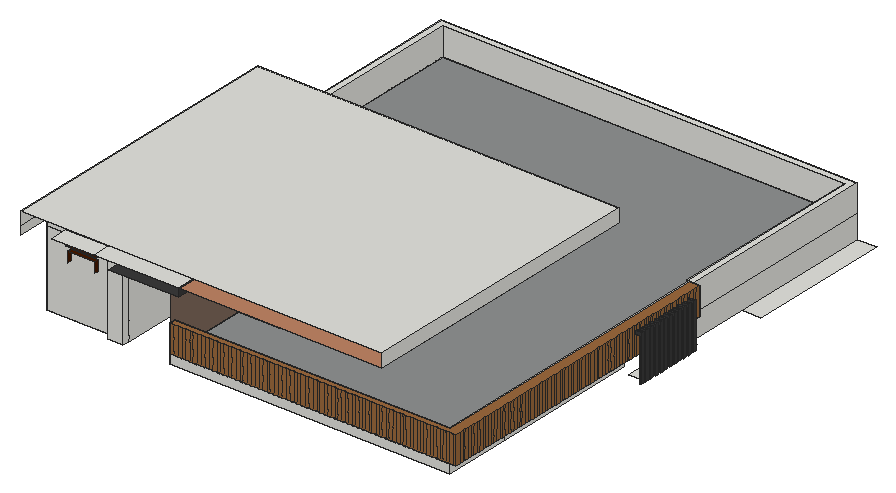
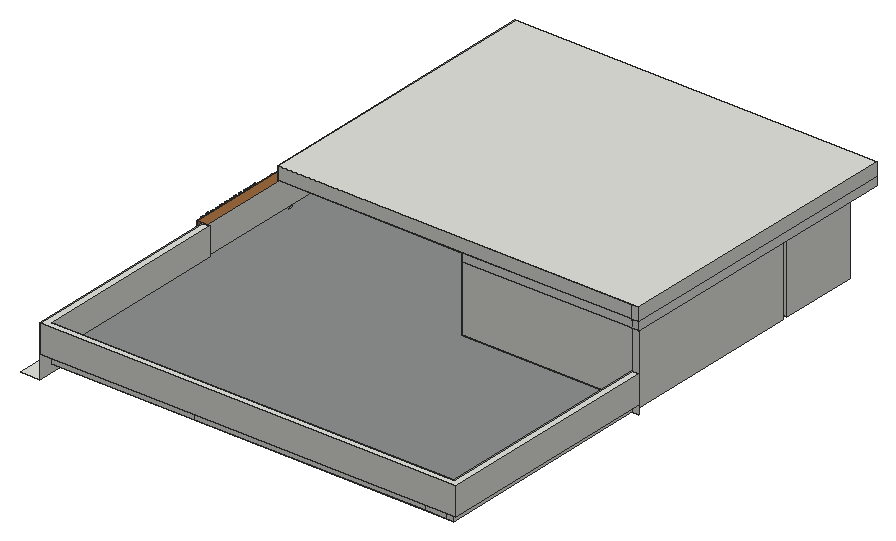
# SketchUp Ruby script. Lengths in inches.
U = 1.inch
M = Sketchup.active_model
def pt(a) = Geom::Point3d.new(a.map { |v| v * U })
def face(e, loops, mat)
  f = e.add_face(loops[0].map { |a| pt(a) })
  loops[1..].each { |l| e.add_face(l.map { |a| pt(a) }).erase! }
  f.material = f.back_material = mat if mat
  f
end
# faces: each face lists its corners as indices into pts; further lists are holes
def faces(e, pts, list, mat = nil) = list.each { |f| face(e, (f[0].is_a?(Array) ? f : [f]).map { |l| l.map { |i| pts[i] } }, mat) }
# xy, xz, yz: faces in a plane at the given z, y or x. An outline is a flat list of corners, or four numbers for a rectangle; further outlines are holes
def ring(l) = l.size == 4 ? [[l[0], l[1]], [l[2], l[1]], [l[2], l[3]], [l[0], l[3]]] : l.each_slice(2).to_a
def flat(e, list, mat, &to3) = list.each { |f| face(e, (f[0].is_a?(Array) ? f : [f]).map { |l| ring(l).map { |u, v| to3.(u, v) } }, mat) }
def xy(e, z, list, mat = nil) = flat(e, list, mat) { |x, y| [x, y, z] }
def xz(e, y, list, mat = nil) = flat(e, list, mat) { |x, z| [x, y, z] }
def yz(e, x, list, mat = nil) = flat(e, list, mat) { |y, z| [x, y, z] }
def lines(e, pts, list) = list.each { |a, b| e.add_line(pt(pts[a]), pt(pts[b])) }
# prism: a flat outline (further loops are holes) pulled along v
def prism(e, loops, v, mat = nil)
  f = face(e, loops, mat); d = Geom::Vector3d.new(v.map { |x| x * U })
  f.pushpull(f.normal.samedirection?(d) ? d.length : -d.length)
end
def box(e, o, s, mat = nil) = prism(e, [[o, [o[0] + s[0], o[1], o[2]], [o[0] + s[0], o[1] + s[1], o[2]], [o[0], o[1] + s[1], o[2]]]], [0, 0, s[2]], mat)
def at(x, y, z, deg = 0) = Geom::Transformation.translation(pt([x, y, z])) * Geom::Transformation.rotation(ORIGIN, Z_AXIS, deg.degrees)
def axes(o, x, y, z) = Geom::Transformation.new([*x, 0, *y, 0, *z, 0, *pt(o).to_a, 1])
def part(name) = M.definitions.add(name)
# library, detail: a bought-in or finely detailed component or shape, given as its bounding box
def library(name, o, s) = part(name).tap { |d| box(d.entities, o, s) }
def detail(e, o, s) = box(e.add_group.entities, o, s)
def put(e, d, t, mat = nil) = e.add_instance(d, t).tap { |i| i.material = mat if mat }
def group(e, t, mat = nil) = e.add_group.tap { |g| g.transformation = t; g.material = mat if mat }.entities
root = M.entities
M.materials.add("[Blacktop Old 02]").color = [143, 145, 145]
M.materials.add("[Color B08]").color = [69, 25, 0]
M.materials.add("[Color E01]").color = [255, 255, 204]
M.materials.add("[Color M07]").color = [58, 58, 58]
M.materials.add("[Granite Brown]").color = [126, 104, 91]
M.materials.add("[Modern Siding]").color = [191, 132, 100]
M.materials.add("[Wood Floor]").color = [155, 105, 61]
xy(root,515.86,[[540,499.48,564.9375,687]])
xy(root,516.1,[[554.5,316.14,556.8125,319.52],[554.5,323.77,556.8125,327.14],[554.5,331.39,556.8125,334.77],[554.5,339.02,556.8125,342.39],[554.5,346.64,556.8125,350.02],
  [554.5,354.27,556.8125,357.64],[554.5,361.89,556.8125,365.27],[554.5,369.52,556.8125,372.89],[554.5,377.14,556.8125,380.52],[554.5,384.77,556.8125,388.14],
  [554.5,392.39,556.8125,395.77],[554.5,400.89,556.8125,404.27]],"[Color M07]")
xy(root,521.1,[[540,316.14,554.5,408.01]])
xy(root,533.5625,[[9,36,18.8125,137.125],[18.8125,36,114.93,137.125],[345.1875,113.4375,345.1875,137.125,351.1875,137.125,351.1875,121.0625,531,121.0625,531,113.4375],[531,113.4375,531.51,137.125],[351.1875,121.0625,531,288],
  [18.8125,137.125,224.375,144.4375],[224.375,137.125,230.375,144.4375],[230.375,137.125,345.1875,144.4375],[345.1875,137.125,345.1875,294,531,294,531,288,351.1875,288,351.1875,137.125],[9,144.4375,18.8125,382.6875],
  [18.8125,144.4375,224.375,382.6875],[224.375,144.4375,224.375,382.6875,18.8125,382.6875,18.8125,388.6875,230.375,388.6875,230.375,144.4375],[230.375,144.4375,230.375,388.6875,18.8125,388.6875,18.8125,678,531,678,531,294,345.1875,294,345.1875,144.4375],[9,388.6875,18.8125,678]])
xy(root,533.5625,[[176.76,25.875,176.76,137.125,345.1875,137.125,345.1875,113.4375,540,113.4375,540,25.875]],"[Wood Floor]")
xy(root,545.5625,[[176.76,25.875,176.76,33.625,534,33.625,534,421.98,540,421.98,540,25.875],[0,388.6875,0,687,540,687,540,421.98,531,421.98,531,678,9,678,9,388.6875]])
xy(root,545.5625,[[176.76,33.625,534,33.625,534,421.98,531,421.98,531,678,9,678,9,388.6875,230.375,388.6875,230.375,137.125,176.76,137.125]],"[Blacktop Old 02]")
xy(root,545.5625,[[540,25.875,548.1875,421.98]],"[Wood Floor]")
xy(root,550.125,[[18.8125,144.4375,224.375,382.6875]])
xy(root,571.13,[[548.25,400.89,554.5,404.27]])
xy(root,571.13,[[547.5625,316.14,554.5,319.52],[548.1875,323.77,554.5,327.14],[548.1875,331.39,554.5,334.77],[548.1875,339.02,554.5,342.39],[548.1875,346.64,554.5,350.02],
  [548.1875,354.27,554.5,357.64],[548.1875,361.89,554.5,365.27],[548.1875,369.52,554.5,372.89],[548.1875,377.14,554.5,380.52],[548.1875,384.77,554.5,388.14],
  [548.1875,392.39,554.5,395.77]],"[Color M07]")
xy(root,575.41,[[548.1875,369.52,556.8125,372.89],[548.1875,377.14,556.8125,380.52],[548.1875,384.77,556.8125,388.14],[548.1875,392.39,556.8125,395.77],[548.25,400.89,556.8125,404.27]],"[Color M07]")
xy(root,575.72,[[547.5625,316.14,556.8125,319.52],[548.1875,323.77,556.8125,327.14],[548.1875,331.39,556.8125,334.77],[548.1875,339.02,556.8125,342.39],[548.1875,346.64,556.8125,350.02],
  [548.1875,354.27,556.8125,357.64],[548.1875,361.89,556.8125,365.27]],"[Color M07]")
xy(root,581.5625,[[0,388.6875,9,388.6875,9,678,531,678,531,421.98,540,421.98,540,687,0,687]])
xy(root,581.5625,[[176.76,25.875,548.1875,25.875,548.1875,421.98,534,421.98,534,33.625,176.76,33.625]],"[Wood Floor]")
xy(root,621.29,[[47.49,22.1875,82.4,27]],"[Color B08]")
xy(root,626.03,[[44.88,22.1875,85.01,27]],"[Color B08]")
xy(root,631.3125,[[94.8,27,114.93,36],[114.93,27,176.76,36],[94.8,36,114.93,137.125],[114.93,36,176.76,137.125],[94.8,137.125,205.99,144.4375],
  [94.8,144.4375,205.99,144.8125]])
xy(root,631.3125,[[114.93,3.875,114.93,27,176.76,27,176.76,137.125,205.99,137.125,205.99,3.875]],"[Color M07]")
xy(root,641.625,[[40.88,3.875,94.8,27],[94.8,3.875,205.99,36],[9,36,94.8,137.125],[94.8,36,205.99,137.125],[94.8,137.125,205.99,144.8125]])
xy(root,641.625,[[205.99,3.875,469.36,137.125],[230.375,137.125,469.36,388.6875]],"[Modern Siding]")
xy(root,658.875,[[0,3.875,469.36,388.6875]])
xz(root,25.875,[[176.76,533.5625,540,545.5625]])
xz(root,25.875,[[176.76,545.5625,181.89,581.5625],[181.89,545.5625,186.89,581.5625],[186.89,545.5625,191.89,581.5625],[191.89,545.5625,196.89,581.5625],[196.89,545.5625,201.89,581.5625],
  [201.89,545.5625,206.89,581.5625],[206.89,545.5625,211.89,581.5625],[211.89,545.5625,216.89,581.5625],[216.89,545.5625,221.89,581.5625],[221.89,545.5625,226.89,581.5625],
  [226.89,545.5625,231.89,581.5625],[231.89,545.5625,236.89,581.5625],[236.89,545.5625,241.89,581.5625],[241.89,545.5625,246.89,581.5625],[246.89,545.5625,251.89,581.5625],
  [251.89,545.5625,256.89,581.5625],[256.89,545.5625,261.89,581.5625],[261.89,545.5625,266.89,581.5625],[266.89,545.5625,271.89,581.5625],[271.89,545.5625,276.89,581.5625],
  [276.89,545.5625,281.89,581.5625],[281.89,545.5625,286.89,581.5625],[286.89,545.5625,291.89,581.5625],[291.89,545.5625,296.89,581.5625],[296.89,545.5625,301.89,581.5625],
  [301.89,545.5625,306.89,581.5625],[306.89,545.5625,311.89,581.5625],[311.89,545.5625,316.89,581.5625],[316.89,545.5625,321.89,581.5625],[321.89,545.5625,326.89,581.5625],
  [326.89,545.5625,331.89,581.5625],[331.89,545.5625,336.89,581.5625],[336.89,545.5625,341.89,581.5625],[341.89,545.5625,346.89,581.5625],[346.89,545.5625,351.89,581.5625],
  [351.89,545.5625,356.89,581.5625],[356.89,545.5625,361.89,581.5625],[361.89,545.5625,366.89,581.5625],[366.89,545.5625,371.89,581.5625],[371.89,545.5625,376.89,581.5625],
  [376.89,545.5625,381.33,581.5625],[381.33,545.5625,385.77,581.5625],[385.77,545.5625,390.2,581.5625],[390.2,545.5625,394.64,581.5625],[394.64,545.5625,399.08,581.5625],
  [399.08,545.5625,403.52,581.5625],[403.52,545.5625,407.95,581.5625],[407.95,545.5625,412.39,581.5625],[412.39,545.5625,416.83,581.5625],[416.83,545.5625,421.27,581.5625],
  [421.27,545.5625,425.7,581.5625],[425.7,545.5625,430.14,581.5625],[430.14,545.5625,434.58,581.5625],[434.58,545.5625,439.02,581.5625],[439.02,545.5625,443.45,581.5625],
  [443.45,545.5625,447.89,581.5625],[447.89,545.5625,452.33,581.5625],[452.33,545.5625,456.77,581.5625],[456.77,545.5625,461.2,581.5625],[461.2,545.5625,465.64,581.5625],
  [465.64,545.5625,470.08,581.5625],[470.08,545.5625,474.52,581.5625],[474.52,545.5625,478.95,581.5625],[478.95,545.5625,483.39,581.5625],[483.39,545.5625,487.83,581.5625],
  [487.83,545.5625,492.27,581.5625],[492.27,545.5625,496.7,581.5625],[496.7,545.5625,501.14,581.5625],[501.14,545.5625,505.58,581.5625],[505.58,545.5625,510.02,581.5625],
  [510.02,545.5625,514.2,581.5625],[514.2,545.5625,518.39,581.5625],[518.39,545.5625,522.58,581.5625],[522.58,545.5625,526.77,581.5625],[526.77,545.5625,530.95,581.5625],
  [530.95,545.5625,535.14,581.5625],[535.14,545.5625,539.33,581.5625],[539.33,545.5625,543.33,581.5625],[543.33,545.5625,548.1875,581.5625]],"[Wood Floor]")
xz(root,27,[[94.8,533.5625,114.93,631.3125]])
xz(root,33.625,[[176.76,545.5625,534,581.5625]])
xz(root,36,[[9,533.5625,114.93,631.3125],[9,631.3125,94.8,641.625]])
xz(root,137.125,[[9,533.5625,22.75,631.3125],[22.75,533.5625,114.93,631.3125],[114.93,533.5625,176.76,631.3125],[176.76,533.5625,224.375,545.5625],[224.375,533.5625,230.375,545.5625],
  [531,533.5625,531.51,545.5625],[9,631.3125,22.75,641.625],[22.75,631.3125,94.8,641.625]])
xz(root,137.125,[[176.76,545.5625,230.375,545.5625,230.375,641.625,205.99,641.625,205.99,631.3125,176.76,631.3125]],"[Color E01]")
xz(root,144.4375,[[9,533.5625,9,631.3125,224.375,631.3125,224.375,550.125,18.8125,550.125,18.8125,533.5625],[18.8125,533.5625,224.375,550.125],[9,631.3125,94.8,641.625],[205.99,631.3125,224.375,641.625]])
xz(root,144.8125,[[94.8,631.3125,205.99,641.625]])
xz(root,316.14,[[554.5,516.1,556.8125,516.1,556.8125,575.72,547.5625,575.72,547.5625,571.13,554.5,571.13]],"[Color M07]")
xz(root,319.52,[[554.5,516.1,554.5,571.13,547.5625,571.13,547.5625,575.72,556.8125,575.72,556.8125,516.1]],"[Color M07]")
xz(root,323.77,[[554.5,516.1,556.8125,516.1,556.8125,575.72,548.1875,575.72,548.1875,571.13,554.5,571.13]],"[Color M07]")
xz(root,327.14,[[554.5,516.1,554.5,571.13,548.1875,571.13,548.1875,575.72,556.8125,575.72,556.8125,516.1]],"[Color M07]")
xz(root,331.39,[[554.5,516.1,556.8125,516.1,556.8125,575.72,548.1875,575.72,548.1875,571.13,554.5,571.13]],"[Color M07]")
xz(root,334.77,[[554.5,516.1,554.5,571.13,548.1875,571.13,548.1875,575.72,556.8125,575.72,556.8125,516.1]],"[Color M07]")
xz(root,339.02,[[554.5,516.1,556.8125,516.1,556.8125,575.72,548.1875,575.72,548.1875,571.13,554.5,571.13]],"[Color M07]")
xz(root,342.39,[[554.5,516.1,554.5,571.13,548.1875,571.13,548.1875,575.72,556.8125,575.72,556.8125,516.1]],"[Color M07]")
xz(root,346.64,[[554.5,516.1,556.8125,516.1,556.8125,575.72,548.1875,575.72,548.1875,571.13,554.5,571.13]],"[Color M07]")
xz(root,350.02,[[554.5,516.1,554.5,571.13,548.1875,571.13,548.1875,575.72,556.8125,575.72,556.8125,516.1]],"[Color M07]")
xz(root,354.27,[[554.5,516.1,556.8125,516.1,556.8125,575.72,548.1875,575.72,548.1875,571.13,554.5,571.13]],"[Color M07]")
xz(root,357.64,[[554.5,516.1,554.5,571.13,548.1875,571.13,548.1875,575.72,556.8125,575.72,556.8125,516.1]],"[Color M07]")
xz(root,361.89,[[554.5,516.1,556.8125,516.1,556.8125,575.72,548.1875,575.72,548.1875,571.13,554.5,571.13]],"[Color M07]")
xz(root,365.27,[[554.5,516.1,554.5,571.13,548.1875,571.13,548.1875,575.72,556.8125,575.72,556.8125,516.1]],"[Color M07]")
xz(root,369.52,[[554.5,516.1,556.8125,516.1,556.8125,575.41,548.1875,575.41,548.1875,571.13,554.5,571.13]],"[Color M07]")
xz(root,372.89,[[554.5,516.1,554.5,571.13,548.1875,571.13,548.1875,575.41,556.8125,575.41,556.8125,516.1]],"[Color M07]")
xz(root,377.14,[[554.5,516.1,556.8125,516.1,556.8125,575.41,548.1875,575.41,548.1875,571.13,554.5,571.13]],"[Color M07]")
xz(root,380.52,[[554.5,516.1,554.5,571.13,548.1875,571.13,548.1875,575.41,556.8125,575.41,556.8125,516.1]],"[Color M07]")
xz(root,382.6875,[[9,533.5625,18.8125,533.5625,18.8125,550.125,224.375,550.125,224.375,631.3125,9,631.3125],[18.8125,533.5625,224.375,550.125],[9,631.3125,224.375,641.625]])
xz(root,384.77,[[554.5,516.1,556.8125,516.1,556.8125,575.41,548.1875,575.41,548.1875,571.13,554.5,571.13]],"[Color M07]")
xz(root,388.14,[[554.5,516.1,554.5,571.13,548.1875,571.13,548.1875,575.41,556.8125,575.41,556.8125,516.1]],"[Color M07]")
xz(root,388.6875,[[0,533.5625,9,545.5625],[9,533.5625,18.8125,545.5625],[18.8125,533.5625,230.375,545.5625],[0,545.5625,9,581.5625],[9,545.5625,230.375,631.3125],
  [0,581.5625,9,631.3125],[0,631.3125,9,641.625],[9,631.3125,230.375,641.625],[0,641.625,9,658.875],[9,641.625,469.36,658.875]])
xz(root,392.39,[[554.5,516.1,556.8125,516.1,556.8125,575.41,548.1875,575.41,548.1875,571.13,554.5,571.13]],"[Color M07]")
xz(root,395.77,[[554.5,516.1,554.5,571.13,548.1875,571.13,548.1875,575.41,556.8125,575.41,556.8125,516.1]],"[Color M07]")
xz(root,400.89,[[554.5,516.1,556.8125,516.1,556.8125,575.41,548.25,575.41,548.25,571.13,554.5,571.13]],"[Color M07]")
xz(root,404.27,[[554.5,516.1,554.5,571.13,548.25,571.13,548.25,575.41,556.8125,575.41,556.8125,516.1]],"[Color M07]")
xz(root,421.98,[[531,545.5625,534,581.5625],[534,545.5625,540,581.5625]])
xz(root,421.98,[[540,545.5625,548.1875,581.5625]],"[Wood Floor]")
xz(root,678,[[9,533.5625,18.8125,545.5625],[18.8125,533.5625,45.875,545.5625],[45.875,533.5625,345.75,545.5625],[345.75,533.5625,531,545.5625],[9,545.5625,531,581.5625]])
xz(root,687,[[0,545.5625,540,581.5625]])
yz(root,0,[[388.6875,545.5625,687,581.5625],[3.875,631.3125,388.6875,641.625],[3.875,641.625,388.6875,658.875]])
yz(root,9,[[36,533.5625,137.125,631.3125],[144.4375,533.5625,382.6875,631.3125],[388.6875,533.5625,678,545.5625],[388.6875,545.5625,678,581.5625],[36,631.3125,137.125,641.625]])
yz(root,18.8125,[[144.4375,533.5625,382.6875,550.125]])
yz(root,47.49,[[22.1875,607.67,27,621.29]],"[Color B08]")
yz(root,82.4,[[22.1875,607.67,27,621.29]],"[Color B08]")
yz(root,94.8,[[27,631.3125,36,641.625],[36,631.3125,137.125,641.625],[137.125,631.3125,144.4375,641.625],[144.4375,631.3125,144.8125,641.625],[144.4375,641.625,144.8125,648.6875]])
yz(root,114.93,[[27,533.5625,36,631.3125],[36,533.5625,137.125,631.3125]])
yz(root,176.76,[[25.875,533.5625,27,545.5625],[27,533.5625,137.125,545.5625],[25.875,545.5625,27,581.5625],[27,545.5625,33.625,581.5625]])
yz(root,176.76,[[33.625,545.5625,137.125,545.5625,137.125,631.3125,27,631.3125,27,581.5625,33.625,581.5625]],"[Granite Brown]")
yz(root,205.99,[[137.125,631.3125,144.4375,641.625],[144.4375,631.3125,144.8125,641.625]])
yz(root,205.99,[[3.875,631.3125,137.125,641.625]],"[Color M07]")
yz(root,224.375,[[144.4375,533.5625,382.6875,550.125],[144.4375,550.125,382.6875,631.3125],[144.4375,631.3125,382.6875,641.625]])
yz(root,230.375,[[137.125,533.5625,144.4375,545.5625],[144.4375,533.5625,388.6875,545.5625]])
yz(root,230.375,[[137.125,545.5625,388.6875,641.625]],"[Color E01]")
yz(root,469.36,[[3.875,641.625,388.6875,658.875]])
yz(root,531,[[288,533.5625,294,545.5625],[421.98,545.5625,678,581.5625]])
yz(root,534,[[33.625,545.5625,421.98,581.5625]])
yz(root,540,[[421.98,515.86,687,545.5625],[25.875,533.5625,113.4375,545.5625],[113.4375,533.5625,308.13,545.5625],[421.98,545.5625,687,581.5625]])
yz(root,547.5625,[[316.14,571.13,319.52,575.72]])
yz(root,548.1875,[[25.875,545.5625,31.59,581.5625],[31.59,545.5625,36.22,581.5625],[36.22,545.5625,40.84,581.5625],[40.84,545.5625,45.47,581.5625],[45.47,545.5625,50.09,581.5625],
  [50.09,545.5625,54.72,581.5625],[54.72,545.5625,59.34,581.5625],[59.34,545.5625,63.97,581.5625],[63.97,545.5625,68.59,581.5625],[68.59,545.5625,73.22,581.5625],
  [73.22,545.5625,77.84,581.5625],[77.84,545.5625,82.47,581.5625],[82.47,545.5625,87.09,581.5625],[87.09,545.5625,91.72,581.5625],[91.72,545.5625,96.34,581.5625],
  [96.34,545.5625,100.97,581.5625],[100.97,545.5625,105.59,581.5625],[105.59,545.5625,110.22,581.5625],[110.22,545.5625,114.84,581.5625],[114.84,545.5625,119.47,581.5625],
  [119.47,545.5625,124.09,581.5625],[124.09,545.5625,128.72,581.5625],[128.72,545.5625,133.34,581.5625],[133.34,545.5625,137.97,581.5625],[137.97,545.5625,142.59,581.5625],
  [142.59,545.5625,147.22,581.5625],[147.22,545.5625,151.84,581.5625],[151.84,545.5625,156.47,581.5625],[156.47,545.5625,161.09,581.5625],[161.09,545.5625,165.72,581.5625],
  [165.72,545.5625,170.34,581.5625],[170.34,545.5625,174.97,581.5625],[174.97,545.5625,179.59,581.5625],[179.59,545.5625,184.22,581.5625],[184.22,545.5625,188.84,581.5625],
  [188.84,545.5625,193.47,581.5625],[193.47,545.5625,198.09,581.5625],[198.09,545.5625,202.72,581.5625],[202.72,545.5625,207.34,581.5625],[207.34,545.5625,211.97,581.5625],
  [211.97,545.5625,216.59,581.5625],[216.59,545.5625,221.22,581.5625],[221.22,545.5625,225.84,581.5625],[225.84,545.5625,230.47,581.5625],[230.47,545.5625,235.09,581.5625],
  [235.09,545.5625,239.72,581.5625],[239.72,545.5625,244.34,581.5625],[244.34,545.5625,248.97,581.5625],[248.97,545.5625,253.59,581.5625],[253.59,545.5625,258.22,581.5625],
  [258.22,545.5625,262.84,581.5625],[262.84,545.5625,267.47,581.5625],[267.47,545.5625,272.09,581.5625],[272.09,545.5625,276.72,581.5625],[276.72,545.5625,281.34,581.5625],
  [281.34,545.5625,285.97,581.5625],[285.97,545.5625,290.59,581.5625],[290.59,545.5625,295.22,581.5625],[295.22,545.5625,299.09,581.5625],[299.09,545.5625,302.97,581.5625],
  [302.97,545.5625,306.84,581.5625],[306.84,545.5625,310.72,581.5625],[310.72,545.5625,314.59,581.5625],[314.59,545.5625,318.47,581.5625],[318.47,545.5625,322.34,581.5625],
  [322.34,545.5625,326.22,545.5625,326.22,571.13,323.77,571.13,323.77,575.72,326.22,575.72,326.22,581.5625,322.34,581.5625],[326.22,545.5625,330.09,545.5625,330.09,581.5625,326.22,581.5625,326.22,575.72,327.14,575.72,327.14,571.13,326.22,571.13],[330.09,545.5625,333.97,545.5625,333.97,571.13,331.39,571.13,331.39,575.72,333.97,575.72,333.97,581.5625,330.09,581.5625],[333.97,545.5625,337.84,545.5625,337.84,581.5625,333.97,581.5625,333.97,575.72,334.77,575.72,334.77,571.13,333.97,571.13],[337.84,545.5625,341.72,545.5625,341.72,571.13,339.02,571.13,339.02,575.72,341.72,575.72,341.72,581.5625,337.84,581.5625],
  [341.72,545.5625,345.59,545.5625,345.59,581.5625,341.72,581.5625,341.72,575.72,342.39,575.72,342.39,571.13,341.72,571.13],[345.59,545.5625,349.47,545.5625,349.47,571.13,346.64,571.13,346.64,575.72,349.47,575.72,349.47,581.5625,345.59,581.5625],[349.47,545.5625,353.34,545.5625,353.34,581.5625,349.47,581.5625,349.47,575.72,350.02,575.72,350.02,571.13,349.47,571.13],[[353.34,545.5625,358.09,581.5625],[354.27,571.13,357.64,575.72]],[358.09,545.5625,362.84,545.5625,362.84,571.13,361.89,571.13,361.89,575.72,362.84,575.72,362.84,581.5625,358.09,581.5625],
  [362.84,545.5625,367.59,545.5625,367.59,581.5625,362.84,581.5625,362.84,575.72,365.27,575.72,365.27,571.13,362.84,571.13],[367.59,545.5625,372.34,545.5625,372.34,571.13,369.52,571.13,369.52,575.41,372.34,575.41,372.34,581.5625,367.59,581.5625],[372.34,545.5625,377.09,545.5625,377.09,581.5625,372.34,581.5625,372.34,575.41,372.89,575.41,372.89,571.13,372.34,571.13],[[377.09,545.5625,381.84,581.5625],[377.14,571.13,380.52,575.41]],[381.84,545.5625,386.59,545.5625,386.59,571.13,384.77,571.13,384.77,575.41,386.59,575.41,386.59,581.5625,381.84,581.5625],
  [386.59,545.5625,391.34,545.5625,391.34,581.5625,386.59,581.5625,386.59,575.41,388.14,575.41,388.14,571.13,386.59,571.13],[[391.34,545.5625,396.09,581.5625],[392.39,571.13,395.77,575.41]],[396.09,545.5625,400.84,581.5625],[400.84,545.5625,405.59,581.5625],[405.59,545.5625,410.34,581.5625],
  [410.34,545.5625,415.09,581.5625],[415.09,545.5625,419.84,581.5625],[419.84,545.5625,421.98,581.5625]],"[Wood Floor]")
yz(root,548.25,[[400.89,571.13,404.27,575.41]])
yz(root,554.5,[[316.14,516.1,319.52,521.1],[323.77,516.1,327.14,521.1],[331.39,516.1,334.77,521.1],[339.02,516.1,342.39,521.1],[346.64,516.1,350.02,521.1],
  [354.27,516.1,357.64,521.1],[361.89,516.1,365.27,521.1],[369.52,516.1,372.89,521.1],[377.14,516.1,380.52,521.1],[384.77,516.1,388.14,521.1],
  [392.39,516.1,395.77,521.1],[400.89,516.1,404.27,521.1]])
yz(root,554.5,[[316.14,521.1,319.52,571.13],[323.77,521.1,327.14,571.13],[331.39,521.1,334.77,571.13],[339.02,521.1,342.39,571.13],[346.64,521.1,350.02,571.13],
  [354.27,521.1,357.64,571.13],[361.89,521.1,365.27,571.13],[369.52,521.1,372.89,571.13],[377.14,521.1,380.52,571.13],[384.77,521.1,388.14,571.13],
  [392.39,521.1,395.77,571.13],[400.89,521.1,404.27,571.13]],"[Color M07]")
yz(root,556.8125,[[316.14,516.1,319.52,575.72],[323.77,516.1,327.14,575.72],[331.39,516.1,334.77,575.72],[339.02,516.1,342.39,575.72],[346.64,516.1,350.02,575.72],
  [354.27,516.1,357.64,575.72],[361.89,516.1,365.27,575.72],[369.52,516.1,372.89,575.41],[377.14,516.1,380.52,575.41],[384.77,516.1,388.14,575.41],
  [392.39,516.1,395.77,575.41],[400.89,516.1,404.27,575.41]],"[Color M07]")
p = [[18.8125,27,533.5625],[18.8125,36,533.5625],[18.8125,678,533.5625],[18.8125,687,533.5625],[351.1875,121.0625,533.5625],[351.1875,121.0625,545.5625],
  [345.1875,113.4375,533.5625],[345.1875,113.4375,545.5625],[531,113.4375,533.5625],[531,113.4375,545.5625],[531,121.0625,533.5625],[531,121.0625,545.5625],
  [351.1875,288,533.5625],[351.1875,288,545.5625],[345.1875,294,533.5625],[345.1875,294,545.5625],[345.1875,137.125,533.5625],[345.1875,137.125,545.5625],
  [9,43.8125,641.625],[9,43.8125,648.6875],[9,36,641.625],[9,36,648.6875],[22.75,137.125,641.625],[22.75,137.125,648.6875],
  [9,382.6875,641.625],[9,382.6875,648.6875],[224.375,382.6875,641.625],[224.375,382.6875,648.6875],[205.99,144.4375,641.625],[205.99,144.4375,648.6875],
  [205.99,137.125,641.625],[205.99,137.125,648.6875],[205.99,144.8125,641.625],[205.99,144.8125,648.6875],[9,137.125,641.625],[9,137.125,648.6875],
  [548.1875,326.22,575.72],[548.1875,326.22,571.13],[548.1875,333.97,575.72],[548.1875,333.97,571.13],[548.1875,341.72,575.72],[548.1875,341.72,571.13],
  [548.1875,349.47,575.72],[548.1875,349.47,571.13],[548.1875,362.84,575.72],[548.1875,362.84,571.13],[548.1875,372.34,575.41],[548.1875,372.34,571.13],
  [548.1875,386.59,575.41],[548.1875,386.59,571.13]]
lines(root,p,[[0,1],[2,3],[4,5],[6,7],[8,9],[10,11],[12,13],[14,15],[16,17],[18,19],[20,21],[22,23],
  [24,25],[26,27],[28,29],[30,31],[32,33],[34,35],[36,37],[38,39],[40,41],[42,43],[44,45],[46,47],
  [48,49]])
